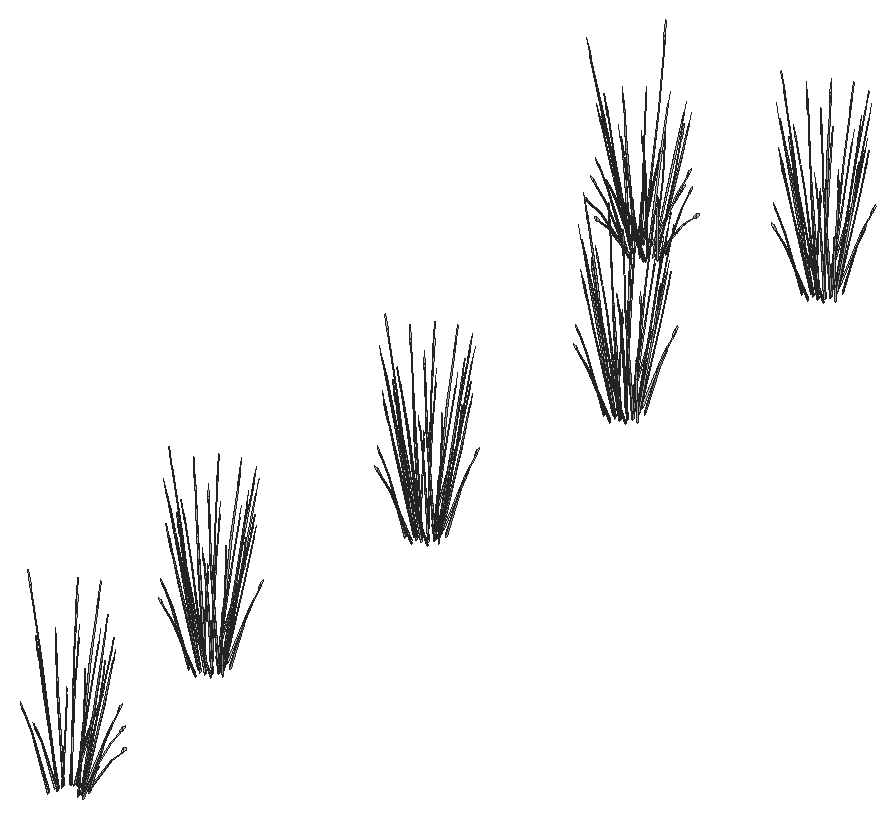
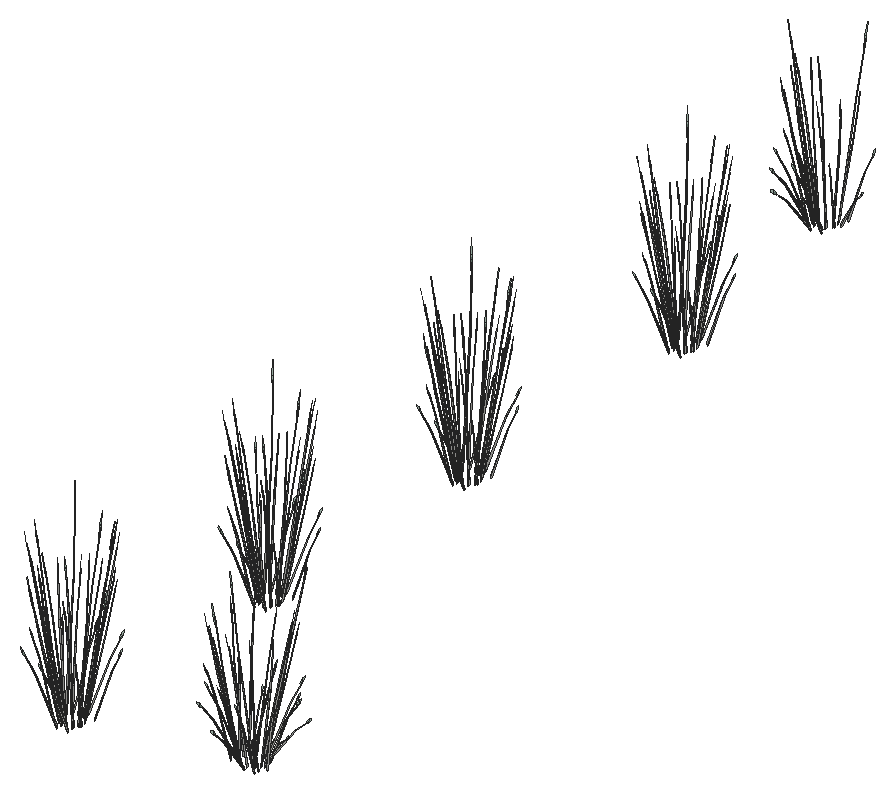
# SketchUp Ruby script. Lengths in inches.
U = 1.inch
M = Sketchup.active_model
def pt(a) = Geom::Point3d.new(a.map { |v| v * U })
def face(e, loops, mat)
  f = e.add_face(loops[0].map { |a| pt(a) })
  loops[1..].each { |l| e.add_face(l.map { |a| pt(a) }).erase! }
  f.material = f.back_material = mat if mat
  f
end
# faces: each face lists its corners as indices into pts; further lists are holes
def faces(e, pts, list, mat = nil) = list.each { |f| face(e, (f[0].is_a?(Array) ? f : [f]).map { |l| l.map { |i| pts[i] } }, mat) }
# xy, xz, yz: faces in a plane at the given z, y or x. An outline is a flat list of corners, or four numbers for a rectangle; further outlines are holes
def ring(l) = l.size == 4 ? [[l[0], l[1]], [l[2], l[1]], [l[2], l[3]], [l[0], l[3]]] : l.each_slice(2).to_a
def flat(e, list, mat, &to3) = list.each { |f| face(e, (f[0].is_a?(Array) ? f : [f]).map { |l| ring(l).map { |u, v| to3.(u, v) } }, mat) }
def xy(e, z, list, mat = nil) = flat(e, list, mat) { |x, y| [x, y, z] }
def xz(e, y, list, mat = nil) = flat(e, list, mat) { |x, z| [x, y, z] }
def yz(e, x, list, mat = nil) = flat(e, list, mat) { |y, z| [x, y, z] }
def lines(e, pts, list) = list.each { |a, b| e.add_line(pt(pts[a]), pt(pts[b])) }
# prism: a flat outline (further loops are holes) pulled along v
def prism(e, loops, v, mat = nil)
  f = face(e, loops, mat); d = Geom::Vector3d.new(v.map { |x| x * U })
  f.pushpull(f.normal.samedirection?(d) ? d.length : -d.length)
end
def box(e, o, s, mat = nil) = prism(e, [[o, [o[0] + s[0], o[1], o[2]], [o[0] + s[0], o[1] + s[1], o[2]], [o[0], o[1] + s[1], o[2]]]], [0, 0, s[2]], mat)
def at(x, y, z, deg = 0) = Geom::Transformation.translation(pt([x, y, z])) * Geom::Transformation.rotation(ORIGIN, Z_AXIS, deg.degrees)
def axes(o, x, y, z) = Geom::Transformation.new([*x, 0, *y, 0, *z, 0, *pt(o).to_a, 1])
def part(name) = M.definitions.add(name)
# library, detail: a bought-in or finely detailed component or shape, given as its bounding box
def library(name, o, s) = part(name).tap { |d| box(d.entities, o, s) }
def detail(e, o, s) = box(e.add_group.entities, o, s)
def put(e, d, t, mat = nil) = e.add_instance(d, t).tap { |i| i.material = mat if mat }
def group(e, t, mat = nil) = e.add_group.tap { |g| g.transformation = t; g.material = mat if mat }.entities
root = M.entities
M.materials.add("LightPink_Translucent").color = [175, 214, 192]
M.materials["LightPink_Translucent"].alpha = 0.75
c1 = part("blade")
p = [[2.15,0.21,22],[0,0.17,0],[0.09,0.45,0],[2.18,0.31,22],[2.29,0.31,22],[0.38,0.45,0],
  [2.48,0.24,33],[2.49,0.24,33],[2.48,0.22,33]]
faces(c1.entities,p,[[0,1,2,3],[4,5,2,3],[6,3,4,7],[8,0,3,6]])
c2 = part("seeds")
p = [[0.3,-0.1,1.38],[-0.01,-0.03,1.59],[-0.01,-0.03,0.03],[0.14,-0.07,-0.07],[0.29,-0.03,3],[0.15,0.01,3.11]]
faces(c2.entities,p,[[0,1,2,3],[1,0,4,5]],"LightPink_Translucent")
c3 = part("blade with seeds")
put(c3.entities,c1,at(0,0,0))
put(c3.entities,c2,axes([2.4,0.25,30.99],[1.5799,-0.05474,1.17369],[-0.12525,1.92788,0.29478],[-0.07173,-0.02425,1.56792]))
put(root,c3,axes([498.03,368.78,141.55],[0.02689,0.05422,1.61419],[-0.17884,0.44816,-0.15253],[-0.14891,-0.01053,0.28566]))
put(root,c3,axes([502.39,370.7,141.57],[0.2829,0.21722,0.05852],[-0.1647,0.30933,0.46065],[0.0907,-0.10001,0.70242]))
put(root,c3,axes([503.22,371.17,141.56],[0.06244,-0.0731,1.59199],[-0.03959,-0.48785,-0.25177],[0.14934,-0.07786,0.12768]))
put(root,c3,axes([499.13,369.9,142.18],[-0.02206,0.52527,-0.12283],[-0.41777,-0.01436,-0.68176],[-0.1609,-0.03649,1.03593]))
put(root,c3,axes([498.5,370.88,141.57],[-0.15135,-0.35217,0.05852],[0.27599,-0.17238,0.46065],[-0.12166,0.03401,0.70242]))
put(root,c3,axes([502.43,371.91,141.57],[0.15135,0.35217,0.05852],[-0.27599,0.17238,0.46065],[0.12166,-0.03401,0.70242]))
put(root,c3,axes([497.85,370.76,141.56],[-0.07171,0.06058,1.59199],[-0.02817,0.48891,-0.25177],[-0.15815,0.04916,0.12768]))
put(root,c3,axes([502.4,371.78,141.57],[-0.11642,0.47094,0.43682],[-0.38276,-0.16104,0.36018],[0.15052,-0.0283,0.9039]))
put(root,c3,axes([502.78,373.26,141.55],[-0.03402,-0.04854,1.61419],[0.11476,-0.47555,-0.15253],[0.14844,-0.01722,0.28566]))
put(root,c3,axes([498.55,372.09,141.57],[-0.2829,-0.21722,0.05852],[0.1647,-0.30933,0.46065],[-0.0907,0.10001,0.70242]))
put(root,c3,axes([498.37,371.61,141.55],[0.05392,0.00141,1.61419],[0.23787,0.40958,-0.15253],[-0.0849,0.14227,0.28566]))
put(root,c3,axes([501.94,372.98,141.57],[-0.02075,0.39276,0.05852],[-0.31333,-0.01077,0.46065],[0.12002,0.0411,0.70242]))
put(root,c3,axes([502.46,373.37,141.56],[0.08863,-0.00461,1.59199],[0.25616,-0.38966,-0.25177],[0.15528,0.06024,0.12768]))
put(root,c3,axes([499.1,373.11,141.57],[-0.33864,-0.02407,0.05852],[0.00928,-0.3634,0.46065],[-0.03543,0.13921,0.70242]))
put(root,c3,axes([499.21,373.14,141.57],[-0.29344,-0.35241,0.43682],[0.31162,-0.30393,0.36018],[-0.05413,0.16534,0.9039]))
put(root,c3,axes([501.0625,373.62,141.57],[-0.18729,0.32811,0.05852],[-0.26671,-0.19103,0.46065],[0.08623,0.10519,0.70242]))
put(root,c3,axes([501.08,374.55,141.55],[0.00338,-0.06243,1.61419],[0.3624,-0.25923,-0.15253],[0.11916,0.1041,0.28566]))
put(root,c3,axes([500.02,373.67,141.57],[-0.30365,0.17554,0.05852],[-0.14862,-0.3201,0.46065],[0.02932,0.1411,0.70242]))
put(root,c3,axes([500.13,373.64,141.57],[-0.40605,-0.13503,0.43682],[0.13885,-0.44393,0.36018],[0.0244,0.17458,0.9039]))
put(root,c3,axes([499.45,373.36,141.56],[0.00753,0.10253,1.59199],[0.34598,0.28122,-0.25177],[-0.04567,0.18237,0.12768]))
put(root,c3,axes([498.82,374.43,141.55],[0.03899,-0.04322,1.61419],[0.41791,0.09454,-0.15253],[0.0267,0.17023,0.28566]))
put(root,c3,axes([500.65,374.78,141.56],[0.06783,0.06632,1.59199],[0.4161,-0.08489,-0.25177],[0.07889,0.16641,0.12768]))
put(root,c3,axes([492.64,412.16,141.46],[-0.01194,0.061,1.61419],[-0.39348,0.18869,-0.15253],[-0.10328,-0.12486,0.28566]))
put(root,c3,axes([494.83,413.39,141.46],[-0.04444,0.03543,1.61419],[-0.3995,-0.17081,-0.15253],[-0.00289,-0.17299,0.28566]))
put(root,c3,axes([493.36,413.37,141.48],[0.40605,0.13503,0.43682],[-0.13885,0.44393,0.36018],[-0.0244,-0.17458,0.9039]))
put(root,c3,axes([493.46,413.33,141.47],[0.30365,-0.17554,0.05852],[0.14862,0.3201,0.46065],[-0.02932,-0.1411,0.70242]))
put(root,c3,axes([492.35,413.47,141.48],[0.40986,-0.11853,0.43682],[0.07113,0.46497,0.36018],[-0.09639,-0.13704,0.9039]))
put(root,c3,axes([492.42,413.38,141.47],[0.18729,-0.32811,0.05852],[0.26671,0.19103,0.46065],[-0.08623,-0.10519,0.70242]))
put(root,c3,axes([494.39,413.89,141.47],[0.33864,0.02407,0.05852],[-0.00928,0.3634,0.46065],[0.03543,-0.13921,0.70242]))
put(root,c3,axes([494.97,415.01,142.11],[-0.42693,-0.31898,-0.12394],[0.24596,-0.46194,-0.6879],[0.12062,-0.16057,1.04526]))
put(root,c3,axes([495.99,414.89,141.46],[-0.05338,-0.00892,1.61419],[-0.19372,-0.43976,-0.15253],[0.09903,-0.12941,0.28566]))
put(root,c3,axes([491.52,414.15,141.48],[0.30385,-0.34034,0.43682],[0.26205,0.36143,0.36018],[-0.14256,-0.06278,0.9039]))
put(root,c3,axes([491.54,414.03,141.47],[0.02075,-0.39276,0.05852],[0.31333,0.01077,0.46065],[-0.12002,-0.0411,0.70242]))
put(root,c3,axes([490.59,413,141.46],[0.02689,0.05422,1.61419],[-0.17884,0.44816,-0.15253],[-0.14891,-0.01053,0.28566]))
put(root,c3,axes([494.94,414.91,141.47],[0.2829,0.21722,0.05852],[-0.1647,0.30933,0.46065],[0.0907,-0.10001,0.70242]))
put(root,c3,axes([491.69,414.11,142.08],[-0.02206,0.52527,-0.12283],[-0.41777,-0.01436,-0.68176],[-0.1609,-0.03649,1.03593]))
put(root,c3,axes([491.0625,415.1,141.47],[-0.15135,-0.35217,0.05852],[0.27599,-0.17238,0.46065],[-0.12166,0.03401,0.70242]))
put(root,c3,axes([494.99,416.12,141.47],[0.15135,0.35217,0.05852],[-0.27599,0.17238,0.46065],[0.12166,-0.03401,0.70242]))
put(root,c3,axes([494.96,415.99,141.48],[-0.11642,0.47094,0.43682],[-0.38276,-0.16104,0.36018],[0.15052,-0.0283,0.9039]))
put(root,c3,axes([495.34,417.48,141.46],[-0.03402,-0.04854,1.61419],[0.11476,-0.47555,-0.15253],[0.14844,-0.01722,0.28566]))
put(root,c3,axes([491.18,416.39,141.48],[-0.1022,-0.47536,0.43682],[0.4009,-0.0825,0.36018],[-0.11815,0.1118,0.9039]))
put(root,c3,axes([491.1,416.3,141.47],[-0.2829,-0.21722,0.05852],[0.1647,-0.30933,0.46065],[-0.0907,0.10001,0.70242]))
put(root,c3,axes([490.93,415.82,141.46],[0.05392,0.00141,1.61419],[0.23787,0.40958,-0.15253],[-0.0849,0.14227,0.28566]))
put(root,c3,axes([494.5,417.1875,141.47],[-0.02075,0.39276,0.05852],[-0.31333,-0.01077,0.46065],[0.12002,0.0411,0.70242]))
put(root,c3,axes([494.53,417.0625,141.48],[-0.30385,0.34034,0.43682],[-0.26205,-0.36143,0.36018],[0.14256,0.06278,0.9039]))
put(root,c3,axes([491.66,417.32,141.47],[-0.33864,-0.02407,0.05852],[0.00928,-0.3634,0.46065],[-0.03543,0.13921,0.70242]))
put(root,c3,axes([491.77,417.36,141.48],[-0.29344,-0.35241,0.43682],[0.31162,-0.30393,0.36018],[-0.05413,0.16534,0.9039]))
put(root,c3,axes([493.62,417.84,141.47],[-0.18729,0.32811,0.05852],[-0.26671,-0.19103,0.46065],[0.08623,0.10519,0.70242]))
put(root,c3,axes([493.7,417.74,141.48],[-0.40986,0.11853,0.43682],[-0.07113,-0.46497,0.36018],[0.09639,0.13704,0.9039]))
put(root,c3,axes([493.64,418.76,141.46],[0.00338,-0.06243,1.61419],[0.3624,-0.25923,-0.15253],[0.11916,0.1041,0.28566]))
put(root,c3,axes([492.58,417.88,141.47],[-0.30365,0.17554,0.05852],[-0.14862,-0.3201,0.46065],[0.02932,0.1411,0.70242]))
put(root,c3,axes([492.6875,417.85,141.48],[-0.40605,-0.13503,0.43682],[0.13885,-0.44393,0.36018],[0.0244,0.17458,0.9039]))
put(root,c3,axes([491.375,418.65,141.46],[0.03899,-0.04322,1.61419],[0.41791,0.09454,-0.15253],[0.0267,0.17023,0.28566]))
put(root,c3,axes([492.64,465.73,141.46],[-0.01194,0.061,1.61419],[-0.39348,0.18869,-0.15253],[-0.10328,-0.12486,0.28566]))
put(root,c3,axes([494.83,466.97,141.46],[-0.04444,0.03543,1.61419],[-0.3995,-0.17081,-0.15253],[-0.00289,-0.17299,0.28566]))
put(root,c3,axes([493.36,466.9375,141.48],[0.40605,0.13503,0.43682],[-0.13885,0.44393,0.36018],[-0.0244,-0.17458,0.9039]))
put(root,c3,axes([493.46,466.91,141.47],[0.30365,-0.17554,0.05852],[0.14862,0.3201,0.46065],[-0.02932,-0.1411,0.70242]))
put(root,c3,axes([492.35,467.05,141.48],[0.40986,-0.11853,0.43682],[0.07113,0.46497,0.36018],[-0.09639,-0.13704,0.9039]))
put(root,c3,axes([492.42,466.95,141.47],[0.18729,-0.32811,0.05852],[0.26671,0.19103,0.46065],[-0.08623,-0.10519,0.70242]))
put(root,c3,axes([494.39,467.47,141.47],[0.33864,0.02407,0.05852],[-0.00928,0.3634,0.46065],[0.03543,-0.13921,0.70242]))
put(root,c3,axes([494.97,468.58,142.11],[-0.42693,-0.31898,-0.12394],[0.24596,-0.46194,-0.6879],[0.12062,-0.16057,1.04526]))
put(root,c3,axes([495.99,468.46,141.46],[-0.05338,-0.00892,1.61419],[-0.19372,-0.43976,-0.15253],[0.09903,-0.12941,0.28566]))
put(root,c3,axes([491.52,467.73,141.48],[0.30385,-0.34034,0.43682],[0.26205,0.36143,0.36018],[-0.14256,-0.06278,0.9039]))
put(root,c3,axes([491.54,467.6,141.47],[0.02075,-0.39276,0.05852],[0.31333,0.01077,0.46065],[-0.12002,-0.0411,0.70242]))
put(root,c3,axes([490.59,466.57,141.46],[0.02689,0.05422,1.61419],[-0.17884,0.44816,-0.15253],[-0.14891,-0.01053,0.28566]))
put(root,c3,axes([494.94,468.49,141.47],[0.2829,0.21722,0.05852],[-0.1647,0.30933,0.46065],[0.0907,-0.10001,0.70242]))
put(root,c3,axes([491.69,467.6875,142.08],[-0.02206,0.52527,-0.12283],[-0.41777,-0.01436,-0.68176],[-0.1609,-0.03649,1.03593]))
put(root,c3,axes([491.0625,468.67,141.47],[-0.15135,-0.35217,0.05852],[0.27599,-0.17238,0.46065],[-0.12166,0.03401,0.70242]))
put(root,c3,axes([494.99,469.69,141.47],[0.15135,0.35217,0.05852],[-0.27599,0.17238,0.46065],[0.12166,-0.03401,0.70242]))
put(root,c3,axes([494.96,469.57,141.48],[-0.11642,0.47094,0.43682],[-0.38276,-0.16104,0.36018],[0.15052,-0.0283,0.9039]))
put(root,c3,axes([495.34,471.05,141.46],[-0.03402,-0.04854,1.61419],[0.11476,-0.47555,-0.15253],[0.14844,-0.01722,0.28566]))
put(root,c3,axes([491.18,469.97,141.48],[-0.1022,-0.47536,0.43682],[0.4009,-0.0825,0.36018],[-0.11815,0.1118,0.9039]))
put(root,c3,axes([491.1,469.875,141.47],[-0.2829,-0.21722,0.05852],[0.1647,-0.30933,0.46065],[-0.0907,0.10001,0.70242]))
put(root,c3,axes([490.93,469.4,141.46],[0.05392,0.00141,1.61419],[0.23787,0.40958,-0.15253],[-0.0849,0.14227,0.28566]))
put(root,c3,axes([494.5,470.76,141.47],[-0.02075,0.39276,0.05852],[-0.31333,-0.01077,0.46065],[0.12002,0.0411,0.70242]))
put(root,c3,axes([494.53,470.64,141.48],[-0.30385,0.34034,0.43682],[-0.26205,-0.36143,0.36018],[0.14256,0.06278,0.9039]))
put(root,c3,axes([491.66,470.9,141.47],[-0.33864,-0.02407,0.05852],[0.00928,-0.3634,0.46065],[-0.03543,0.13921,0.70242]))
put(root,c3,axes([491.77,470.93,141.48],[-0.29344,-0.35241,0.43682],[0.31162,-0.30393,0.36018],[-0.05413,0.16534,0.9039]))
put(root,c3,axes([493.62,471.41,141.47],[-0.18729,0.32811,0.05852],[-0.26671,-0.19103,0.46065],[0.08623,0.10519,0.70242]))
put(root,c3,axes([493.7,471.32,141.48],[-0.40986,0.11853,0.43682],[-0.07113,-0.46497,0.36018],[0.09639,0.13704,0.9039]))
put(root,c3,axes([493.64,472.34,141.46],[0.00338,-0.06243,1.61419],[0.3624,-0.25923,-0.15253],[0.11916,0.1041,0.28566]))
put(root,c3,axes([492.58,471.46,141.47],[-0.30365,0.17554,0.05852],[-0.14862,-0.3201,0.46065],[0.02932,0.1411,0.70242]))
put(root,c3,axes([492.6875,471.42,141.48],[-0.40605,-0.13503,0.43682],[0.13885,-0.44393,0.36018],[0.0244,0.17458,0.9039]))
put(root,c3,axes([491.375,472.22,141.46],[0.03899,-0.04322,1.61419],[0.41791,0.09454,-0.15253],[0.0267,0.17023,0.28566]))
put(root,c3,axes([492.64,514.9375,141.46],[-0.01194,0.061,1.61419],[-0.39348,0.18869,-0.15253],[-0.10328,-0.12486,0.28566]))
put(root,c3,axes([494.83,516.18,141.46],[-0.04444,0.03543,1.61419],[-0.3995,-0.17081,-0.15253],[-0.00289,-0.17299,0.28566]))
put(root,c3,axes([493.36,516.15,141.48],[0.40605,0.13503,0.43682],[-0.13885,0.44393,0.36018],[-0.0244,-0.17458,0.9039]))
put(root,c3,axes([493.46,516.12,141.47],[0.30365,-0.17554,0.05852],[0.14862,0.3201,0.46065],[-0.02932,-0.1411,0.70242]))
put(root,c3,axes([492.35,516.26,141.48],[0.40986,-0.11853,0.43682],[0.07113,0.46497,0.36018],[-0.09639,-0.13704,0.9039]))
put(root,c3,axes([492.42,516.16,141.47],[0.18729,-0.32811,0.05852],[0.26671,0.19103,0.46065],[-0.08623,-0.10519,0.70242]))
put(root,c3,axes([494.39,516.68,141.47],[0.33864,0.02407,0.05852],[-0.00928,0.3634,0.46065],[0.03543,-0.13921,0.70242]))
put(root,c3,axes([494.97,517.79,142.11],[-0.42693,-0.31898,-0.12394],[0.24596,-0.46194,-0.6879],[0.12062,-0.16057,1.04526]))
put(root,c3,axes([495.99,517.67,141.46],[-0.05338,-0.00892,1.61419],[-0.19372,-0.43976,-0.15253],[0.09903,-0.12941,0.28566]))
put(root,c3,axes([491.52,516.93,141.48],[0.30385,-0.34034,0.43682],[0.26205,0.36143,0.36018],[-0.14256,-0.06278,0.9039]))
put(root,c3,axes([491.54,516.81,141.47],[0.02075,-0.39276,0.05852],[0.31333,0.01077,0.46065],[-0.12002,-0.0411,0.70242]))
put(root,c3,axes([490.59,515.78,141.46],[0.02689,0.05422,1.61419],[-0.17884,0.44816,-0.15253],[-0.14891,-0.01053,0.28566]))
put(root,c3,axes([494.94,517.7,141.47],[0.2829,0.21722,0.05852],[-0.1647,0.30933,0.46065],[0.0907,-0.10001,0.70242]))
put(root,c3,axes([491.69,516.9,142.08],[-0.02206,0.52527,-0.12283],[-0.41777,-0.01436,-0.68176],[-0.1609,-0.03649,1.03593]))
put(root,c3,axes([491.0625,517.88,141.47],[-0.15135,-0.35217,0.05852],[0.27599,-0.17238,0.46065],[-0.12166,0.03401,0.70242]))
put(root,c3,axes([494.99,518.9,141.47],[0.15135,0.35217,0.05852],[-0.27599,0.17238,0.46065],[0.12166,-0.03401,0.70242]))
put(root,c3,axes([494.96,518.78,141.48],[-0.11642,0.47094,0.43682],[-0.38276,-0.16104,0.36018],[0.15052,-0.0283,0.9039]))
put(root,c3,axes([495.34,520.26,141.46],[-0.03402,-0.04854,1.61419],[0.11476,-0.47555,-0.15253],[0.14844,-0.01722,0.28566]))
put(root,c3,axes([491.18,519.18,141.48],[-0.1022,-0.47536,0.43682],[0.4009,-0.0825,0.36018],[-0.11815,0.1118,0.9039]))
put(root,c3,axes([491.1,519.09,141.47],[-0.2829,-0.21722,0.05852],[0.1647,-0.30933,0.46065],[-0.0907,0.10001,0.70242]))
put(root,c3,axes([490.93,518.61,141.46],[0.05392,0.00141,1.61419],[0.23787,0.40958,-0.15253],[-0.0849,0.14227,0.28566]))
put(root,c3,axes([494.5,519.97,141.47],[-0.02075,0.39276,0.05852],[-0.31333,-0.01077,0.46065],[0.12002,0.0411,0.70242]))
put(root,c3,axes([494.53,519.85,141.48],[-0.30385,0.34034,0.43682],[-0.26205,-0.36143,0.36018],[0.14256,0.06278,0.9039]))
put(root,c3,axes([491.66,520.11,141.47],[-0.33864,-0.02407,0.05852],[0.00928,-0.3634,0.46065],[-0.03543,0.13921,0.70242]))
put(root,c3,axes([491.77,520.14,141.48],[-0.29344,-0.35241,0.43682],[0.31162,-0.30393,0.36018],[-0.05413,0.16534,0.9039]))
put(root,c3,axes([493.62,520.62,141.47],[-0.18729,0.32811,0.05852],[-0.26671,-0.19103,0.46065],[0.08623,0.10519,0.70242]))
put(root,c3,axes([493.7,520.53,141.48],[-0.40986,0.11853,0.43682],[-0.07113,-0.46497,0.36018],[0.09639,0.13704,0.9039]))
put(root,c3,axes([493.64,521.54,141.46],[0.00338,-0.06243,1.61419],[0.3624,-0.25923,-0.15253],[0.11916,0.1041,0.28566]))
put(root,c3,axes([492.58,520.67,141.47],[-0.30365,0.17554,0.05852],[-0.14862,-0.3201,0.46065],[0.02932,0.1411,0.70242]))
put(root,c3,axes([492.6875,520.63,141.48],[-0.40605,-0.13503,0.43682],[0.13885,-0.44393,0.36018],[0.0244,0.17458,0.9039]))
put(root,c3,axes([491.375,521.43,141.46],[0.03899,-0.04322,1.61419],[0.41791,0.09454,-0.15253],[0.0267,0.17023,0.28566]))
put(root,c3,axes([463.08,557.29,141.56],[-0.0731,-0.06244,1.59199],[-0.48785,0.03959,-0.25177],[-0.07786,-0.14934,0.12768]))
put(root,c3,axes([465.27,558.05,141.56],[-0.00461,-0.08863,1.59199],[-0.38966,-0.25616,-0.25177],[0.06024,-0.15528,0.12768]))
put(root,c3,axes([465.17,557.74,141.55],[-0.04854,0.03402,1.61419],[-0.47555,-0.11476,-0.15253],[-0.01722,-0.14844,0.28566]))
put(root,c3,axes([462.58,557.08,141.55],[-0.00892,0.05338,1.61419],[-0.43976,0.19372,-0.15253],[-0.12941,-0.09903,0.28566]))
put(root,c3,axes([463.81,558.09,141.57],[0.35217,-0.15135,0.05852],[0.17238,0.27599,0.46065],[-0.03401,-0.12166,0.70242]))
put(root,c3,axes([462.6,558.13,141.57],[0.21722,-0.2829,0.05852],[0.30933,0.1647,0.46065],[-0.10001,-0.0907,0.70242]))
put(root,c3,axes([462.7,558.1,142.21],[-0.31898,0.42693,-0.12394],[-0.46194,-0.24596,-0.6879],[-0.16057,-0.12062,1.04526]))
put(root,c3,axes([464.88,558.57,141.57],[0.39276,0.02075,0.05852],[-0.01077,0.31333,0.46065],[0.0411,-0.12002,0.70242]))
put(root,c3,axes([461.48,557.98,141.56],[-0.10283,-0.00314,1.59199],[-0.32739,0.31434,-0.25177],[-0.17468,-0.06423,0.12768]))
put(root,c3,axes([466.45,559.43,141.55],[-0.06243,-0.00338,1.61419],[-0.25923,-0.3624,-0.15253],[0.1041,-0.11916,0.28566]))
put(root,c3,axes([461.58,558.68,141.57],[0.02407,-0.33864,0.05852],[0.3634,0.00928,0.46065],[-0.13921,-0.03543,0.70242]))
put(root,c3,axes([465.52,559.45,141.57],[0.32811,0.18729,0.05852],[-0.19103,0.26671,0.46065],[0.10519,-0.08623,0.70242]))
put(root,c3,axes([466.6875,559.87,141.56],[0.06632,-0.06783,1.59199],[-0.08489,-0.4161,-0.25177],[0.16641,-0.07889,0.12768]))
put(root,c3,axes([461.08,558.24,141.55],[0.03543,0.04444,1.61419],[-0.17081,0.3995,-0.15253],[-0.17299,0.00289,0.28566]))
put(root,c3,axes([461.02,559.61,141.57],[-0.17554,-0.30365,0.05852],[0.3201,-0.14862,0.46065],[-0.1411,0.02932,0.70242]))
put(root,c3,axes([465.57,560.49,141.57],[0.17554,0.30365,0.05852],[-0.3201,0.14862,0.46065],[0.1411,-0.02932,0.70242]))
put(root,c3,axes([466.34,561.7,141.55],[-0.04322,-0.03899,1.61419],[0.09454,-0.41791,-0.15253],[0.17023,-0.0267,0.28566]))
put(root,c3,axes([460.71,560,141.56],[-0.07805,0.05782,1.59199],[0.00664,0.42244,-0.25177],[-0.1789,0.05494,0.12768]))
put(root,c3,axes([465.26,561.0625,141.56],[0.10253,-0.00753,1.59199],[0.28122,-0.34598,-0.25177],[0.18237,0.04567,0.12768]))
put(root,c3,axes([492.64,563.99,141.46],[-0.01194,0.061,1.61419],[-0.39348,0.18869,-0.15253],[-0.10328,-0.12486,0.28566]))
put(root,c3,axes([461.07,560.65,141.57],[-0.32811,-0.18729,0.05852],[0.19103,-0.26671,0.46065],[-0.10519,0.08623,0.70242]))
put(root,c3,axes([494.83,565.22,141.46],[-0.04444,0.03543,1.61419],[-0.3995,-0.17081,-0.15253],[-0.00289,-0.17299,0.28566]))
put(root,c3,axes([493.36,565.2,141.48],[0.40605,0.13503,0.43682],[-0.13885,0.44393,0.36018],[-0.0244,-0.17458,0.9039]))
put(root,c3,axes([459.85,560.43,141.55],[0.061,0.01194,1.61419],[0.18869,0.39348,-0.15253],[-0.12486,0.10328,0.28566]))
put(root,c3,axes([493.46,565.16,141.47],[0.30365,-0.17554,0.05852],[0.14862,0.3201,0.46065],[-0.02932,-0.1411,0.70242]))
put(root,c3,axes([465.01,561.41,141.57],[-0.02407,0.33864,0.05852],[-0.3634,-0.00928,0.46065],[0.13921,0.03543,0.70242]))
put(root,c3,axes([492.35,565.3,141.48],[0.40986,-0.11853,0.43682],[0.07113,0.46497,0.36018],[-0.09639,-0.13704,0.9039]))
put(root,c3,axes([492.42,565.21,141.47],[0.18729,-0.32811,0.05852],[0.26671,0.19103,0.46065],[-0.08623,-0.10519,0.70242]))
put(root,c3,axes([494.39,565.72,141.47],[0.33864,0.02407,0.05852],[-0.00928,0.3634,0.46065],[0.03543,-0.13921,0.70242]))
put(root,c3,axes([494.97,566.84,142.11],[-0.42693,-0.31898,-0.12394],[0.24596,-0.46194,-0.6879],[0.12062,-0.16057,1.04526]))
put(root,c3,axes([463.51,562.15,141.55],[0.00141,-0.05392,1.61419],[0.40958,-0.23787,-0.15253],[0.14227,0.0849,0.28566]))
put(root,c3,axes([461.72,561.53,141.57],[-0.39276,-0.02075,0.05852],[0.01077,-0.31333,0.46065],[-0.0411,0.12002,0.70242]))
put(root,c3,axes([463.99,561.97,141.57],[-0.21722,0.2829,0.05852],[-0.30933,-0.1647,0.46065],[0.10001,0.0907,0.70242]))
put(root,c3,axes([495.99,566.72,141.46],[-0.05338,-0.00892,1.61419],[-0.19372,-0.43976,-0.15253],[0.09903,-0.12941,0.28566]))
put(root,c3,axes([462.79,562.01,141.57],[-0.35217,0.15135,0.05852],[-0.17238,-0.27599,0.46065],[0.03401,0.12166,0.70242]))
put(root,c3,axes([460.73,561.58,141.56],[-0.01188,0.08813,1.59199],[0.33715,0.30658,-0.25177],[-0.08826,0.14498,0.12768]))
put(root,c3,axes([461.8,561.38,142.18],[0.52527,0.02206,-0.12283],[-0.01436,0.41777,-0.68176],[-0.03649,0.1609,1.03593]))
put(root,c3,axes([491.52,565.98,141.48],[0.30385,-0.34034,0.43682],[0.26205,0.36143,0.36018],[-0.14256,-0.06278,0.9039]))
put(root,c3,axes([491.54,565.86,141.47],[0.02075,-0.39276,0.05852],[0.31333,0.01077,0.46065],[-0.12002,-0.0411,0.70242]))
put(root,c3,axes([490.59,564.83,141.46],[0.02689,0.05422,1.61419],[-0.17884,0.44816,-0.15253],[-0.14891,-0.01053,0.28566]))
put(root,c3,axes([460.6875,562.48,141.55],[0.05422,-0.02689,1.61419],[0.44816,0.17884,-0.15253],[-0.01053,0.14891,0.28566]))
put(root,c3,axes([494.94,566.75,141.47],[0.2829,0.21722,0.05852],[-0.1647,0.30933,0.46065],[0.0907,-0.10001,0.70242]))
put(root,c3,axes([462.67,562.67,141.56],[0.06058,0.07171,1.59199],[0.48891,0.02817,-0.25177],[0.04916,0.15815,0.12768]))
put(root,c3,axes([491.69,565.95,142.08],[-0.02206,0.52527,-0.12283],[-0.41777,-0.01436,-0.68176],[-0.1609,-0.03649,1.03593]))
put(root,c3,axes([491.0625,566.93,141.47],[-0.15135,-0.35217,0.05852],[0.27599,-0.17238,0.46065],[-0.12166,0.03401,0.70242]))
put(root,c3,axes([494.99,567.95,141.47],[0.15135,0.35217,0.05852],[-0.27599,0.17238,0.46065],[0.12166,-0.03401,0.70242]))
put(root,c3,axes([494.96,567.83,141.48],[-0.11642,0.47094,0.43682],[-0.38276,-0.16104,0.36018],[0.15052,-0.0283,0.9039]))
put(root,c3,axes([495.34,569.31,141.46],[-0.03402,-0.04854,1.61419],[0.11476,-0.47555,-0.15253],[0.14844,-0.01722,0.28566]))
put(root,c3,axes([491.18,568.23,141.48],[-0.1022,-0.47536,0.43682],[0.4009,-0.0825,0.36018],[-0.11815,0.1118,0.9039]))
put(root,c3,axes([491.1,568.13,141.47],[-0.2829,-0.21722,0.05852],[0.1647,-0.30933,0.46065],[-0.0907,0.10001,0.70242]))
put(root,c3,axes([490.93,567.66,141.46],[0.05392,0.00141,1.61419],[0.23787,0.40958,-0.15253],[-0.0849,0.14227,0.28566]))
put(root,c3,axes([494.5,569.02,141.47],[-0.02075,0.39276,0.05852],[-0.31333,-0.01077,0.46065],[0.12002,0.0411,0.70242]))
put(root,c3,axes([494.53,568.9,141.48],[-0.30385,0.34034,0.43682],[-0.26205,-0.36143,0.36018],[0.14256,0.06278,0.9039]))
put(root,c3,axes([491.66,569.16,141.47],[-0.33864,-0.02407,0.05852],[0.00928,-0.3634,0.46065],[-0.03543,0.13921,0.70242]))
put(root,c3,axes([491.77,569.1875,141.48],[-0.29344,-0.35241,0.43682],[0.31162,-0.30393,0.36018],[-0.05413,0.16534,0.9039]))
put(root,c3,axes([493.62,569.67,141.47],[-0.18729,0.32811,0.05852],[-0.26671,-0.19103,0.46065],[0.08623,0.10519,0.70242]))
put(root,c3,axes([493.7,569.58,141.48],[-0.40986,0.11853,0.43682],[-0.07113,-0.46497,0.36018],[0.09639,0.13704,0.9039]))
put(root,c3,axes([493.64,570.59,141.46],[0.00338,-0.06243,1.61419],[0.3624,-0.25923,-0.15253],[0.11916,0.1041,0.28566]))
put(root,c3,axes([492.58,569.72,141.47],[-0.30365,0.17554,0.05852],[-0.14862,-0.3201,0.46065],[0.02932,0.1411,0.70242]))
put(root,c3,axes([492.6875,569.68,141.48],[-0.40605,-0.13503,0.43682],[0.13885,-0.44393,0.36018],[0.0244,0.17458,0.9039]))
put(root,c3,axes([491.375,570.48,141.46],[0.03899,-0.04322,1.61419],[0.41791,0.09454,-0.15253],[0.0267,0.17023,0.28566]))
